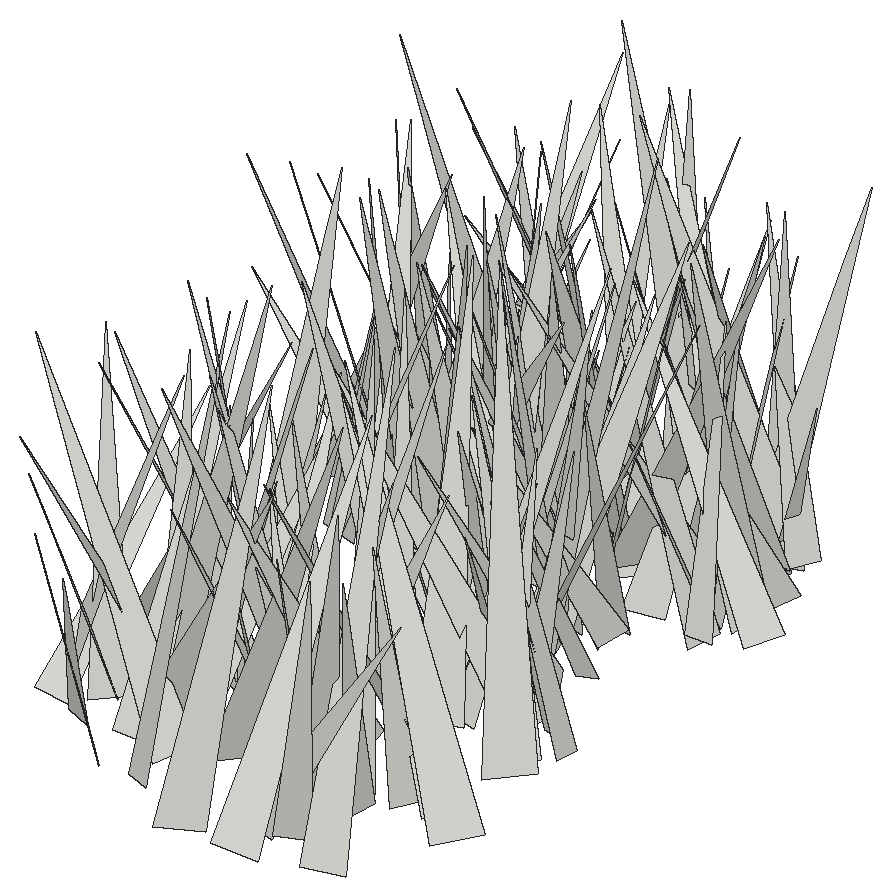
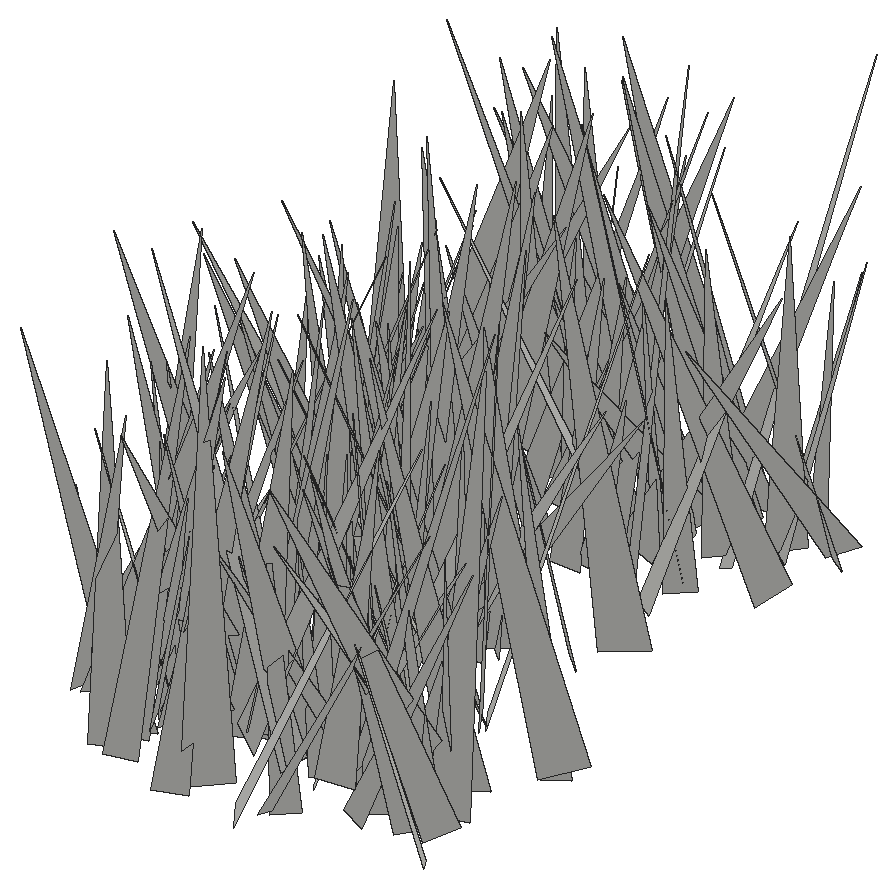
# SketchUp Ruby script. Lengths in inches.
U = 1.inch
M = Sketchup.active_model
def pt(a) = Geom::Point3d.new(a.map { |v| v * U })
def face(e, loops, mat)
  f = e.add_face(loops[0].map { |a| pt(a) })
  loops[1..].each { |l| e.add_face(l.map { |a| pt(a) }).erase! }
  f.material = f.back_material = mat if mat
  f
end
# faces: each face lists its corners as indices into pts; further lists are holes
def faces(e, pts, list, mat = nil) = list.each { |f| face(e, (f[0].is_a?(Array) ? f : [f]).map { |l| l.map { |i| pts[i] } }, mat) }
# xy, xz, yz: faces in a plane at the given z, y or x. An outline is a flat list of corners, or four numbers for a rectangle; further outlines are holes
def ring(l) = l.size == 4 ? [[l[0], l[1]], [l[2], l[1]], [l[2], l[3]], [l[0], l[3]]] : l.each_slice(2).to_a
def flat(e, list, mat, &to3) = list.each { |f| face(e, (f[0].is_a?(Array) ? f : [f]).map { |l| ring(l).map { |u, v| to3.(u, v) } }, mat) }
def xy(e, z, list, mat = nil) = flat(e, list, mat) { |x, y| [x, y, z] }
def xz(e, y, list, mat = nil) = flat(e, list, mat) { |x, z| [x, y, z] }
def yz(e, x, list, mat = nil) = flat(e, list, mat) { |y, z| [x, y, z] }
def lines(e, pts, list) = list.each { |a, b| e.add_line(pt(pts[a]), pt(pts[b])) }
# prism: a flat outline (further loops are holes) pulled along v
def prism(e, loops, v, mat = nil)
  f = face(e, loops, mat); d = Geom::Vector3d.new(v.map { |x| x * U })
  f.pushpull(f.normal.samedirection?(d) ? d.length : -d.length)
end
def box(e, o, s, mat = nil) = prism(e, [[o, [o[0] + s[0], o[1], o[2]], [o[0] + s[0], o[1] + s[1], o[2]], [o[0], o[1] + s[1], o[2]]]], [0, 0, s[2]], mat)
def at(x, y, z, deg = 0) = Geom::Transformation.translation(pt([x, y, z])) * Geom::Transformation.rotation(ORIGIN, Z_AXIS, deg.degrees)
def axes(o, x, y, z) = Geom::Transformation.new([*x, 0, *y, 0, *z, 0, *pt(o).to_a, 1])
def part(name) = M.definitions.add(name)
# library, detail: a bought-in or finely detailed component or shape, given as its bounding box
def library(name, o, s) = part(name).tap { |d| box(d.entities, o, s) }
def detail(e, o, s) = box(e.add_group.entities, o, s)
def put(e, d, t, mat = nil) = e.add_instance(d, t).tap { |i| i.material = mat if mat }
def group(e, t, mat = nil) = e.add_group.tap { |g| g.transformation = t; g.material = mat if mat }.entities
root = M.entities
c1 = part("fur_instance\#9")
p = [[0.8125,0,1.79],[0.67,-0.02,1.48],[0,-0.11,0],[0,0.11,0]]
faces(c1.entities,p,[[0,1,2,3]])
put(root,c1,axes([146.41,46.61,-27.1],[2.86346,-4.49186,1.0378],[-4.60706,-2.8331,0.44926],[-0.16992,1.11803,5.30796]))
put(root,c1,axes([138.79,46.7,-27.1],[-2.84095,-2.72325,0.75235],[-2.80656,2.8428,-0.30791],[0.32453,0.74533,3.9233]))
put(root,c1,axes([145.17,46.39,-27.1],[2.54302,-4.52945,1.06711],[-4.23804,-1.75205,2.66287],[1.92189,2.12978,4.46004]))
put(root,c1,axes([143.4,44.91,-27.1],[5.43285,-3.6045,3.64876],[-4.74936,-5.54221,1.59663],[-1.93634,3.48041,6.32132]))
put(root,c1,axes([136.69,48.41,-27.1],[-0.43336,-3.79274,0.22877],[-3.61563,0.48241,1.14868],[1.16807,0.08612,3.64049]))
put(root,c1,axes([137.43,51.93,-27.1],[-5.00279,-6.48805,0.18943],[-5.66686,4.48249,3.86684],[3.16501,-2.22958,7.22289]))
put(root,c1,axes([145.65,48.75,-27.1],[5.23742,-3.794,0.7561],[-3.79638,-5.28528,-0.22367],[-0.74406,0.26094,6.46336]))
put(root,c1,axes([145.58,44.87,-27.1],[-1.59566,7.05244,0.57454],[6.94745,1.67322,-1.24356],[1.34162,-0.27674,7.12297]))
put(root,c1,axes([146.96,49.14,-27.1],[4.83805,-1.95602,0.87332],[-1.75837,-4.85831,-1.14034],[-1.22345,-0.75248,5.09238]))
put(root,c1,axes([138.8,49.68,-27.1],[2.77166,-6.45652,0.14972],[-5.9267,-2.47813,2.8503],[2.56578,1.25036,6.42219]))
put(root,c1,axes([144.97,49.34,-27.1],[3.60771,1.96245,2.32029],[2.67745,-3.75626,-0.98607],[-1.43745,-2.07119,3.98679]))
put(root,c1,axes([140.375,48.45,-27.1],[-6.66331,2.16551,0.21128],[2.17487,6.60915,0.85019],[-0.06344,-0.87375,6.95459]))
put(root,c1,axes([136.41,50.5,-27.1],[-3.04266,-3.74721,0.50143],[-3.60797,3.07034,1.05183],[1.12942,-0.28668,4.71094]))
put(root,c1,axes([142.25,51.57,-27.1],[-3.9218,-4.42687,0.35438],[-4.07666,3.77609,2.05553],[1.7617,-1.11678,5.54549]))
put(root,c1,axes([148.41,45.6,-27.1],[0.0768,8.17284,0.16546],[8.06568,-0.10268,1.32775],[-1.3295,-0.15078,8.06464]))
put(root,c1,axes([141.87,49.24,-27.1],[6.48225,-3.39085,0.68777],[-3.4557,-6.41712,0.9323],[-0.17042,1.14593,7.25591]))
put(root,c1,axes([140.53,46.45,-27.1],[3.83849,6.3713,1.10198],[6.13828,-3.99344,1.70758],[-2.03209,-0.02789,7.23959]))
put(root,c1,axes([144.49,49.09,-27.1],[1.01992,4.1189,1.46608],[4.23417,-0.55549,-1.38501],[1.0893,-1.69737,4.0109]))
put(root,c1,axes([144.74,52.42,-27.1],[-6.04066,-0.63869,2.51357],[0.73038,5.69455,3.20222],[2.48847,-3.22176,5.16172]))
put(root,c1,axes([148.51,51.32,-27.1],[-2.23247,-5.83337,0.18602],[-5.6892,2.13065,-1.46288],[-1.30221,0.692,6.07224]))
put(root,c1,axes([142.72,50.27,-27.1],[-2.07432,-2.92088,0.84042],[-3.01146,2.11274,-0.09003],[0.41107,0.73854,3.58137]))
put(root,c1,axes([147.82,50.4,-27.1],[-3.6167,2.28369,2.19841],[2.80718,3.85669,0.61192],[1.47241,-1.74341,4.23336]))
put(root,c1,axes([144.92,50.83,-27.1],[1.50784,-3.41822,0.5063],[-3.4457,-1.52893,-0.06057],[-0.26023,0.4385,3.73552]))
put(root,c1,axes([143.4,52.11,-27.1],[1.95168,-6.84621,1.26966],[-6.52036,-2.2596,-2.16121],[-2.44285,0.56154,6.78298]))
put(root,c1,axes([144.15,50.15,-27.1],[4.85202,-3.37562,1.03104],[-3.52041,-4.75453,1.00059],[-0.25408,1.41409,5.82544]))
put(root,c1,axes([134.9,49.71,-27.1],[4.20289,4.66758,0.96744],[4.74909,-3.98911,-1.38552],[0.41036,-1.63927,6.12625]))
put(root,c1,axes([150.39,49.66,-27.1],[-4.97351,5.86998,1.15657],[5.9442,4.67754,1.82131],[-0.6788,-2.04794,7.47498]))
put(root,c1,axes([144.8,48.65,-27.1],[3.51205,7.24819,1.1392],[7.33442,-3.43356,-0.76524],[0.20101,-1.35755,8.01781]))
put(root,c1,axes([144.77,50.04,-27.1],[-7.94923,-1.56442,0.5472],[-1.62855,7.87073,-1.15603],[0.30767,1.24144,8.0188]))
put(root,c1,axes([139.36,51.0625,-27.1],[3.2608,1.42212,0.87051],[1.60342,-3.19897,-0.78016],[-0.45742,-1.07574,3.47082]))
put(root,c1,axes([136.67,49.96,-27.1],[-4.60516,3.74944,1.60687],[3.84875,4.79672,-0.16237],[1.35183,-0.88372,5.93628]))
put(root,c1,axes([140.39,49.5,-27.1],[4.26964,0.47793,1.18834],[0.14194,-4.28676,1.21405],[-1.27296,1.12502,4.1212]))
put(root,c1,axes([138.6,49.83,-27.1],[7.3545,-2.24014,2.18394],[-2.66673,-7.40612,1.38362],[-1.63595,2.00191,7.56257]))
put(root,c1,axes([144.25,50.67,-27.1],[2.31719,-2.3997,1.71249],[-2.74416,-2.55172,0.13746],[-1.07739,1.33819,3.33302]))
put(root,c1,axes([149.03,50.79,-27.1],[-5.22041,4.31379,0.87725],[4.39805,5.05275,1.32586],[-0.18846,-1.57859,6.64105]))
put(root,c1,axes([143.22,50.87,-27.1],[-3.14224,2.77876,1.0294],[2.91205,3.17344,0.32264],[0.54877,-0.92877,4.18224]))
put(root,c1,axes([138.76,48.47,-27.1],[0.11708,7.08162,0.20269],[7.08451,-0.11681,-0.01106],[0.00771,-0.20285,7.08258]))
put(root,c1,axes([146.03,50.17,-27.1],[0.42916,7.00561,1.64499],[7.11073,-0.66598,0.98114],[-1.10544,-1.56418,6.94983]))
put(root,c1,axes([135.26,48.95,-27.1],[-2.44099,4.81015,0.04297],[4.37742,2.2412,-2.21652],[1.99437,0.96814,4.91762]))
put(root,c1,axes([140.65,53.84,-27.1],[-0.18064,-6.52008,0.8881],[-6.57997,0.17015,-0.08916],[-0.06535,0.89016,6.52198]))
put(root,c1,axes([137.96,51.41,-27.1],[3.60386,-3.42869,2.87422],[-4.08632,-4.02533,0.32181],[-1.82182,2.24626,4.96388]))
put(root,c1,axes([138.57,55.16,-27.1],[-4.91582,-6.36103,2.07601],[-5.8042,5.33544,2.60426],[3.32923,-0.09063,7.60565]))
put(root,c1,axes([137.95,53.33,-27.1],[5.79589,4.16761,1.50359],[4.42839,-5.37215,-2.17978],[0.13803,-2.64446,6.79779]))
put(root,c1,axes([137.8125,55.41,-27.1],[-3.98509,-5.15803,0.00595],[-5.07141,3.91953,1.18509],[0.94137,-0.71992,6.40951]))
put(root,c1,axes([140.28,52.74,-27.1],[-1.81659,5.58818,1.87966],[5.39696,0.78429,2.88421],[-2.37355,-2.49359,5.11948]))
put(root,c1,axes([139.4,52.64,-27.1],[1.95895,3.98258,1.69888],[4.26762,-2.09086,-0.01944],[-0.73116,-1.53362,4.43825]))
put(root,c1,axes([135.21,52.4,-27.1],[6.85637,-0.90607,0.05149],[-0.90407,-6.7849,0.99057],[0.07926,0.98874,6.84468]))
put(root,c1,axes([139.62,50.28,-27.1],[-3.68567,4.23937,0.30212],[3.60627,3.33103,-2.74713],[2.24908,1.60613,4.89997]))
put(root,c1,axes([137.53,53.98,-27.1],[-2.45808,3.26284,2.53045],[3.74921,2.99751,-0.22312],[1.72995,-1.86016,4.07903]))
put(root,c1,axes([141.08,51.95,-27.1],[-2.87102,4.68172,0.40163],[4.57171,2.89185,-1.02921],[1.08596,0.20316,5.39463]))
put(root,c1,axes([142.53,54.32,-27.1],[1.52627,-4.48364,1.33128],[-4.39877,-0.90019,2.01128],[1.58937,1.81423,4.28804]))
put(root,c1,axes([141.25,54.89,-27.1],[0.46643,-4.66615,1.44002],[-4.86096,-0.58186,-0.31092],[-0.46655,1.39737,4.67909]))
put(root,c1,axes([144.375,55.51,-27.1],[4.0303,-5.81988,3.12764],[-5.66664,-4.92868,-1.86917],[-3.39741,1.31665,6.82792]))
put(root,c1,axes([149.18,53.7,-27.1],[-6.71454,4.39928,1.56364],[4.39375,6.8803,-0.4901],[1.57912,-0.43767,8.0124]))
put(root,c1,axes([147.71,56.43,-27.1],[-4.43221,4.72995,1.58971],[4.78005,3.41433,3.16821],[-1.43205,-3.24253,5.65503]))
put(root,c1,axes([140.52,54.53,-27.1],[-1.14245,4.14217,0.46464],[4.01441,0.96381,1.27839],[-1.12161,-0.76952,4.10226]))
put(root,c1,axes([140.23,53.22,-27.1],[5.64336,5.1887,0.30355],[5.15395,-5.64438,0.66329],[-0.67191,0.28398,7.63742]))
put(root,c1,axes([148.5625,56.52,-27.1],[-1.63509,-3.83691,0.93062],[-3.94815,1.58786,-0.39017],[-0.00453,1.00909,4.15248]))
put(root,c1,axes([145.66,57.87,-27.1],[-0.82646,-4.24361,0.01629],[-4.06802,0.79698,1.2278],[1.20816,-0.21938,4.14533]))
put(root,c1,axes([148.79,54.63,-27.1],[-4.40287,4.25609,0.42122],[4.26988,4.40886,0.08361],[0.24458,-0.35298,6.12311]))
put(root,c1,axes([146.87,58.99,-27.1],[-4.92711,-3.11526,0.5387],[-2.69685,4.66208,2.29422],[1.64986,-1.68274,5.3589]))
put(root,c1,axes([148.49,54.45,-27.1],[-4.43133,1.84787,0.51045],[1.62369,4.30117,-1.47494],[1.01922,1.18203,4.56901]))
put(root,c1,axes([145.41,54.89,-27.1],[-2.63415,6.93544,1.64719],[7.09873,2.71215,-0.06728],[0.64926,-1.51533,7.41852]))
put(root,c1,axes([147.15,56.875,-27.1],[-4.76846,2.17787,1.48985],[2.383,4.8757,0.4998],[1.13316,-1.08876,5.21838]))
put(root,c1,axes([149.72,55.79,-27.1],[-6.70794,-1.60484,0.19836],[-1.59675,6.44001,-1.8942],[-0.25542,1.88735,6.63204]))
put(root,c1,axes([137.375,56.8125,-27.1],[1.77196,3.84512,1.4323],[4.08534,-1.50774,-1.0065],[0.38272,-1.70823,4.11239]))
put(root,c1,axes([146.46,57.375,-27.1],[0.92533,-3.44435,1.34936],[-3.58141,-1.18238,-0.56215],[-0.92618,1.13092,3.52189]))
put(root,c1,axes([143.45,55.51,-27.1],[-0.40472,6.25604,0.83945],[6.18781,0.22712,1.29072],[-1.24649,-0.90382,6.13481]))
put(root,c1,axes([145.23,56.27,-27.1],[3.77133,0.16267,0.95437],[-0.10228,-3.74984,1.04331],[-0.96272,1.03561,3.6278]))
put(root,c1,axes([144.08,59.74,-27.1],[4.85347,-3.26157,0.26621],[-3.0891,-4.72355,-1.55255],[-1.07988,-1.1468,5.6377]))
put(root,c1,axes([146.98,57.32,-27.1],[4.06657,-2.17936,1.39694],[-2.40276,-4.14574,0.52683],[-0.9632,1.14071,4.58356]))
put(root,c1,axes([145.72,55.51,-27.1],[2.14003,7.20036,0.0672],[7.19519,-2.14104,0.27303],[-0.28086,0.01341,7.50668]))
put(root,c1,axes([136.58,57.83,-27.1],[-2.68799,6.56885,2.98447],[6.8694,3.30396,-1.08507],[2.20641,-2.2839,7.01411]))
put(root,c1,axes([141.82,59.57,-27.1],[7.52805,-0.18805,1.99939],[0.07054,-7.72753,-0.99239],[-2.00698,-0.97696,7.46472]))
put(root,c1,axes([143.22,60.36,-27.1],[-6.0404,2.2493,3.21945],[3.13358,6.3206,1.46334],[2.36747,-2.62704,6.2773]))
put(root,c1,axes([147.16,59.96,-27.1],[-0.83843,-4.56243,0.7415],[-4.45874,0.59959,-1.35228],[-1.2187,0.94513,4.43735]))
put(root,c1,axes([144.71,57.46,-27.1],[-3.134,4.47853,0.59876],[4.43295,3.18866,-0.64743],[0.8745,-0.1137,5.42771]))
put(root,c1,axes([140.36,61.11,-27.1],[1.08245,-7.41016,1.80762],[-7.58562,-1.23679,-0.52762],[-0.7977,1.70574,7.47019]))
put(root,c1,axes([141.34,61.09,-27.1],[1.42395,-7.42701,2.10024],[-7.62151,-1.69014,-0.80943],[-1.21824,1.89264,7.51884]))
put(root,c1,axes([146.28,62.32,-27.1],[3.38656,-3.48151,1.0277],[-2.77448,-3.38882,-2.33752],[-2.3408,-1.02022,4.25743]))
put(root,c1,axes([139.91,60.01,-27.1],[-4.37552,-5.12362,2.64469],[-5.63456,4.50416,-0.59611],[1.22377,2.41912,6.71129]))
put(root,c1,axes([145.33,60.91,-27.1],[-6.26815,-2.22604,2.13273],[-2.17784,6.6177,0.5065],[2.18193,0.21043,6.63238]))
put(root,c1,axes([140.89,60.79,-27.1],[-3.83855,4.56526,0.77541],[4.17711,2.97899,3.13921],[-1.99865,-2.54191,5.07163]))
put(root,c1,axes([137.43,59.3,-27.1],[2.58432,3.47984,0.90101],[3.42396,-2.72089,0.68775],[-1.09434,-0.29537,4.2796]))
put(root,c1,axes([145.52,58.74,-27.1],[6.4283,2.09347,0.22673],[2.03253,-6.35917,1.08941],[-0.55031,0.96716,6.67224]))
put(root,c1,axes([145.21,60.52,-27.1],[5.91491,-0.67607,1.90084],[-0.77835,-6.19702,0.21795],[-1.8613,0.44302,5.94943]))
put(root,c1,axes([145.85,62.93,-27.1],[0.34868,-5.31048,0.36463],[-5.26358,-0.28954,0.81646],[0.79301,0.41316,5.25892]))
put(root,c1,axes([137.14,63.8,-27.1],[-6.21102,-4.85766,0.88936],[-4.64444,6.23147,1.60082],[1.67841,-0.73247,7.72082]))
put(root,c1,axes([144.45,64.03,-28.22],[-6.5639,-4.29471,0.69968],[-4.06333,6.50273,1.7952],[1.55674,-1.13527,7.63588]))
put(root,c1,axes([141.12,60.06,-27.1],[-6.11447,-3.98639,0.59028],[-3.68819,5.10346,-3.73879],[-1.62389,3.41906,6.26894]))
put(root,c1,axes([143.76,60.29,-27.1],[-4.22823,5.63878,0.60494],[5.64653,4.11564,1.10357],[-0.52773,-1.14251,6.96102]))
put(root,c1,axes([144.16,63.45,-27.1],[-4.57132,-4.01454,0.83204],[-3.89365,4.6413,1.00178],[1.28384,-0.21818,6.00082]))
put(root,c1,axes([138.18,63.78,-27.1],[1.13503,-7.67663,0.6742],[-6.50823,-0.58999,4.2389],[4.12651,1.18099,6.50005]))
put(root,c1,axes([139.35,59.78,-27.1],[-4.20767,6.2047,0.57896],[6.20765,4.23458,-0.26697],[0.54635,-0.32858,7.49209]))
put(root,c1,axes([144.33,59.26,-27.1],[3.4696,4.95294,0.18512],[4.68916,-3.35343,1.83583],[-1.60551,0.90933,5.7619]))
put(root,c1,axes([141.11,62.59,-27.1],[5.21956,1.10973,1.69595],[1.36173,-5.39042,-0.66376],[-1.50115,-1.03121,5.29478]))
put(root,c1,axes([140.17,64.52,-27.1],[-4.57477,-6.03245,0.25242],[-6.03633,4.57654,-0.02819],[0.13005,0.21817,7.57088]))
put(root,c1,axes([146.06,58.62,-27.1],[7.29611,1.84526,3.54482],[-0.04664,-7.33917,3.91643],[-3.99607,3.45479,6.4265]))
put(root,c1,axes([134.5,63.76,-28.22],[0.54307,-5.39112,1.14857],[-5.29865,-0.1925,1.60174],[1.51911,1.25582,5.17624]))
put(root,c1,axes([140.59,63.66,-28.22],[6.72646,1.81373,2.96578],[2.30607,-7.16166,-0.85049],[-2.60144,-1.65881,6.91459]))
put(root,c1,axes([144.55,61.13,-27.1],[-2.83058,6.09964,1.95872],[5.76034,3.3604,-2.14023],[2.80369,-0.74599,6.37473]))
put(root,c1,axes([142.11,64.96,-27.1],[2.97455,-6.14482,0.55918],[-6.16848,-2.94679,0.43089],[0.14598,0.69067,6.8133]))
put(root,c1,axes([140.75,63.15,-27.1],[1.70203,4.17643,2.24286],[4.55719,-2.09788,0.44817],[-1.30578,-1.87783,4.48761]))
put(root,c1,axes([143.98,62.23,-27.1],[0.03547,5.69131,1.501],[5.73382,0.30561,-1.29426],[1.32938,-1.46999,5.5423]))
put(root,c1,axes([144.48,62.46,-27.1],[-6.24639,-1.28271,0.8155],[-1.43317,6.11916,-1.35263],[0.50635,1.49608,6.23162]))
put(root,c1,axes([141.22,64.93,-27.1],[5.81845,-0.62274,2.18855],[-0.03101,-6.03017,-1.6334],[-2.27522,-1.51035,5.61909]))
put(root,c1,axes([141.76,63.3,-27.1],[-3.37291,-1.64413,0.77782],[-1.79286,3.28135,-0.83849],[0.30629,1.10194,3.65741]))
put(root,c1,axes([141.93,61.83,-27.1],[-0.24232,8.0833,1.63068],[8.24361,0.27788,-0.15248],[0.20433,-1.625,8.08549]))
put(root,c1,axes([137.36,63.79,-27.1],[-5.46878,-3.64969,2.6695],[-4.02035,5.84198,-0.2491],[2.0696,1.70441,6.57007]))
put(root,c1,axes([137.02,65.34,-28.22],[5.21183,-0.69159,1.00189],[-0.40075,-5.13378,-1.45906],[-1.14955,-1.3458,5.051]))
put(root,c1,axes([138.2,63.49,-28.22],[3.11612,2.14822,0.04863],[2.13222,-3.08072,-0.53874],[0.26618,-0.47091,3.74631]))
put(root,c1,axes([133.34,64.82,-27.1],[5.01421,-5.55154,0.43768],[-5.45899,-4.78379,1.86233],[1.10028,1.565,7.24525]))
put(root,c1,axes([146.52,67.51,-28.22],[-6.99156,-3.62516,0.34789],[-3.32905,6.6672,2.57109],[1.47657,-2.13338,7.444]))
put(root,c1,axes([143.4,63.27,-27.1],[3.40494,2.47984,0.75094],[2.39973,-3.48584,0.63038],[-0.97714,0.08048,4.16483]))
put(root,c1,axes([143.88,63.54,-28.22],[2.11114,4.26728,1.69749],[4.08085,-2.60007,1.46097],[-2.10662,-0.76029,4.53125]))
put(root,c1,axes([137.3,63.77,-27.1],[4.92095,5.18553,0.33695],[5.09859,-4.72846,-1.69263],[1.00379,-1.4039,6.94554]))
put(root,c1,axes([148,64.83,-27.1],[-3.22375,-2.36609,0.00506],[-2.25529,3.0702,-1.21594],[-0.71558,0.9831,3.80952]))
put(root,c1,axes([139.46,65.26,-27.1],[-0.7765,-5.95979,2.50914],[-6.25232,1.3369,1.24057],[1.65027,2.26084,5.88073]))
put(root,c1,axes([148.35,63.86,-27.1],[0.28645,5.00767,1.03913],[5.08565,-0.389,0.47271],[-0.54104,-1.00525,4.99354]))
put(root,c1,axes([143.35,65.36,-28.22],[5.91305,2.63208,1.30513],[2.84881,-5.85376,-1.10147],[-0.71801,-1.54954,6.37799]))
put(root,c1,axes([141.27,64.5625,-27.1],[1.148,3.43718,0.90942],[3.54891,-1.0498,-0.51218],[0.21566,-1.0212,3.58745]))
put(root,c1,axes([149.99,65.01,-27.1],[-4.53112,4.00144,0.54603],[3.94801,4.21612,1.86503],[-0.85024,-1.74745,5.75015]))
put(root,c1,axes([142.72,66.98,-27.1],[-2.91514,-5.53327,1.42514],[-5.42873,3.18122,1.24695],[1.78243,0.63944,6.12864]))
put(root,c1,axes([141.09,66.24,-27.1],[3.87563,-0.57439,1.14349],[-0.32332,-3.96837,-0.89752],[-1.23813,-0.76168,3.81378]))
put(root,c1,axes([140.42,65.34,-28.22],[4.6292,0.17151,0.50537],[0.17521,-4.6565,-0.02456],[-0.5041,-0.0434,4.63231]))
put(root,c1,axes([147.22,67.36,-27.1],[1.68994,-6.65431,0.98946],[-6.7239,-1.70391,0.02495],[-0.21912,0.96522,6.8655]))
put(root,c1,axes([135.6,67.6,-28.22],[0.64901,-7.30772,0.94418],[-7.33385,-0.54888,0.79295],[0.71332,1.00569,7.2935]))
put(root,c1,axes([140.78,65.02,-28.22],[-0.2633,5.21725,2.01289],[5.21535,0.95622,-1.79623],[2.01778,-1.79073,4.90536]))
put(root,c1,axes([141.66,68.48,-27.1],[5.49992,-4.64771,0.52674],[-4.40214,-5.41809,-1.84207],[-1.58109,-1.08206,6.96111]))
put(root,c1,axes([137.22,67.37,-28.22],[3.42862,-3.42654,1.21049],[-3.04602,-3.61734,-1.61199],[-1.98197,-0.36822,4.57144]))
put(root,c1,axes([147.3,65.43,-28.22],[-7.05219,-0.0174,0.36445],[-0.04272,7.04446,-0.49029],[0.36236,0.49184,7.03515]))
put(root,c1,axes([139.93,68.65,-28.22],[-4.13321,-3.41194,0.20507],[-3.07913,3.85633,2.10107],[1.48403,-1.5014,4.93054]))
put(root,c1,axes([143.77,66.04,-27.1],[7.07032,-2.50038,0.22823],[-2.5064,-6.98854,1.08245],[0.14815,1.09629,7.42089]))
put(root,c1,axes([140.6,66.37,-28.22],[-3.23089,-3.2407,0.20186],[-3.09319,2.98531,-1.58167],[-0.98745,1.25194,4.29408]))
put(root,c1,axes([136.15,65.92,-28.22],[1.86303,-6.4471,2.90273],[-6.99316,-1.23765,1.73947],[1.04242,3.21946,6.48153]))
put(root,c1,axes([143.08,67.04,-27.1],[-3.69542,-5.95234,1.80806],[-6.20183,3.68953,-0.52934],[0.48649,1.82006,6.98615]))
put(root,c1,axes([148.42,67.03,-28.22],[-2.94659,-4.28728,0.79485],[-4.35538,2.84813,-0.78348],[-0.2081,1.09651,5.14289]))
put(root,c1,axes([146.64,66.4375,-27.1],[-2.09497,-3.98677,2.51489],[-4.46346,2.56262,0.34425],[1.51546,2.03632,4.49052]))
put(root,c1,axes([137.96,65.73,-27.1],[3.6626,3.70148,0.35684],[3.71844,-3.64024,-0.40601],[0.03906,-0.53912,5.19141]))
put(root,c1,axes([138.32,65.73,-28.22],[2.93854,2.24557,1.05284],[2.03507,-3.11619,0.96641],[-1.41759,0.18132,3.56983]))
put(root,c1,axes([147.68,66.89,-28.22],[-4.77809,0.40303,0.49366],[0.4272,4.79644,0.21897],[0.47289,-0.2608,4.79006]))
put(root,c1,axes([141.6,67.73,-27.1],[5.62437,-1.82953,0.08499],[-1.8284,-5.62476,-0.0835],[-0.10665,-0.05312,5.91386]))
put(root,c1,axes([147.75,68.84,-28.22],[2.95419,-3.46444,1.08183],[-2.95275,-3.10527,-1.88109],[-2.11044,-0.50488,4.14621]))
put(root,c1,axes([141.02,66.91,-28.22],[1.67153,-3.68103,1.97281],[-4.08391,-1.88531,-0.05752],[-0.87388,1.76964,4.04237]))
put(root,c1,axes([136.32,66.71,-28.22],[2.05844,3.54151,1.67651],[3.74882,-2.33096,0.32115],[-1.13989,-1.27062,4.08367]))
put(root,c1,axes([138.6,65.73,-28.22],[1.45638,3.8911,0.37542],[3.87774,-1.48869,0.38679],[-0.49475,-0.21394,4.13668]))
put(root,c1,axes([142.1,69.19,-27.1],[-4.63636,-6.55031,0.51962],[-6.56307,4.58532,-0.75728],[-0.32055,0.86066,7.9893]))
put(root,c1,axes([138.32,68.51,-27.1],[-7.66466,-1.90179,1.421],[-1.79066,7.78455,0.75987],[1.55871,-0.40873,7.86043]))
put(root,c1,axes([147.3125,68.85,-27.1],[-0.33805,-5.61743,0.95415],[-5.65981,0.22074,-0.70569],[-0.6576,0.9879,5.58317]))
put(root,c1,axes([136.26,67.48,-28.22],[2.41252,4.65389,1.89869],[5.02303,-2.30836,-0.72433],[-0.1815,-2.02404,5.19175]))
put(root,c1,axes([140.15,68.07,-28.22],[0.50859,-3.54434,0.97529],[-3.61365,-0.30136,0.78924],[0.67458,1.05784,3.49258]))
put(root,c1,axes([137.42,68.73,-28.22],[0.50493,-3.90237,0.56248],[-3.75126,-0.30094,1.27958],[1.21364,0.69337,3.72104]))
put(root,c1,axes([146.99,68.09,-27.1],[-2.52237,2.99386,0.77548],[2.99232,2.10973,1.58806],[-0.78138,-1.58517,3.57821]))
put(root,c1,axes([143.84,68.22,-28.22],[6.74375,-1.56753,0.95704],[-1.61805,-6.79399,0.27364],[-0.86892,0.48558,6.91813]))
put(root,c1,axes([142.55,66.68,-28.22],[1.32341,3.79294,0.4756],[3.74321,-1.38791,0.65276],[-0.77522,-0.22654,3.9638]))
put(root,c1,axes([143.74,70.31,-28.22],[-4.79038,-5.44103,1.36632],[-5.2062,4.98101,1.5825],[2.08977,-0.06337,7.07448]))
put(root,c1,axes([137.79,69.4375,-28.22],[-1.33885,-4.31341,0.19295],[-4.24788,1.27969,-0.86785],[-0.77346,0.43835,4.43226]))
put(root,c1,axes([137.4,68.46,-27.1],[4.80931,3.10321,2.02961],[3.46778,-4.94111,-0.66234],[-1.31293,-1.68352,5.68513]))
put(root,c1,axes([145.71,68.34,-28.22],[0.99186,4.25892,2.03749],[4.71935,-0.95274,-0.30591],[-0.13232,-2.05608,4.36218]))
put(root,c1,axes([143.3,67.41,-28.22],[-4.74257,5.72398,1.5327],[5.90767,4.72004,0.65254],[0.46105,-1.60076,7.40474]))
put(root,c1,axes([147.29,69.46,-27.1],[-7.26006,2.55391,1.83228],[2.95803,7.11093,1.80912],[1.0629,-2.34529,7.48051]))
put(root,c1,axes([144.82,65.61,-28.22],[-4.70627,4.28235,1.06672],[3.70191,4.67966,-2.45399],[2.40255,1.178,5.87073]))
put(root,c1,axes([143.54,68.06,-27.1],[4.7353,0.6555,1.15241],[0.55235,-4.8611,0.49538],[-1.20525,0.34759,4.75472]))
put(root,c1,axes([138.68,67.43,-28.22],[0.32449,4.79651,0.65441],[4.29347,0.01783,-2.25961],[2.23626,-0.73022,4.24334]))
put(root,c1,axes([140.02,69.49,-27.1],[8.09633,1.85359,0.38508],[1.89305,-7.94545,-1.5559],[-0.02113,-1.6027,8.15877]))
put(root,c1,axes([144.97,70.02,-27.1],[-5.38028,-3.08502,1.66928],[-3.07413,5.61908,0.47644],[1.68926,0.39986,6.18367]))
put(root,c1,axes([146.23,67.74,-27.1],[3.62964,3.56201,0.97293],[3.43547,-3.75775,0.94107],[-1.35352,0.01415,4.99765]))
put(root,c1,axes([139.58,70.43,-28.22],[2.72527,-3.47225,0.02549],[-3.46346,-2.7159,0.33551],[0.24824,0.22715,4.40125]))
put(root,c1,axes([138.33,69.62,-27.1],[1.39978,-5.30319,2.32473],[-5.64349,-1.78474,-0.67328],[-1.29585,2.04412,5.44334]))
put(root,c1,axes([146.63,69.91,-28.22],[3.71508,-1.29272,0.27873],[-1.28155,-3.72443,-0.19222],[-0.32626,-0.0905,3.92887]))
put(root,c1,axes([135.88,68.85,-28.22],[3.16186,-4.77933,2.12939],[-5.21892,-2.70344,1.68164],[0.37303,2.68757,5.47827]))
put(root,c1,axes([136.93,65.98,-28.22],[5.40862,3.75774,0.29196],[3.28966,-4.95573,2.84217],[-1.83956,2.18614,5.94103]))
put(root,c1,axes([144.36,72.4,-27.1],[-0.43827,-6.52973,0.002],[-6.42899,0.43186,1.145],[1.14256,-0.07472,6.44348]))
put(root,c1,axes([133.84,70.0625,-27.1],[3.57334,-4.4658,0.19156],[-4.12422,-3.19939,2.34597],[1.72363,1.60293,5.21618]))
put(root,c1,axes([146.41,68.3125,-27.1],[-6.04879,4.39479,0.23194],[4.40071,6.03643,0.38865],[-0.04117,-0.45072,7.46666]))
put(root,c1,axes([144.76,71.1875,-27.1],[1.52104,-3.59534,0.18519],[-3.58042,-1.53172,-0.32978],[-0.37596,0.04131,3.88989]))
put(root,c1,axes([144.45,69.35,-27.1],[-8.05212,1.79962,1.36323],[1.82873,8.16018,0.02927],[1.32393,-0.32629,8.25072]))
put(root,c1,axes([140.72,71.45,-28.22],[-5.75391,-4.14909,0.07824],[-4.14913,5.75437,0.02082],[0.07564,0.02888,7.0938]))
put(root,c1,axes([146.48,67.74,-27.1],[-5.7713,0.32455,0.04644],[0.28097,5.31808,-2.2482],[0.16895,2.24233,5.3253]))
put(root,c1,axes([141.24,67.33,-28.22],[-5.90287,3.96424,1.22936],[3.5461,5.92766,-2.08769],[2.15678,1.10365,6.7971]))
put(root,c1,axes([134.35,70.26,-28.22],[4.18709,2.7222,0.51054],[2.74144,-3.94162,-1.4666],[0.39441,-1.502,4.77401]))
put(root,c1,axes([136.74,66.42,-28.22],[-5.0261,5.87636,0.71878],[5.2638,4.86732,-2.98524],[2.70938,1.44485,7.13314]))
put(root,c1,axes([143.11,71.6,-28.22],[2.7716,-4.32676,0.73791],[-4.29866,-2.85215,-0.57784],[-0.88707,0.30254,5.10575]))
put(root,c1,axes([138.86,72.33,-27.1],[-4.92347,-1.39259,0.14711],[-1.23579,4.5738,1.93769],[0.65861,-1.82825,4.73553]))
put(root,c1,axes([146.26,70.51,-28.22],[-1.98157,5.41612,3.08152],[6.10168,2.34277,-0.19399],[1.26474,-2.81671,5.76397]))
put(root,c1,axes([147.97,69.42,-27.1],[-5.43325,1.77797,0.85582],[1.73658,5.49897,-0.39929],[0.93695,0.1182,5.7028]))
put(root,c1,axes([146.22,69.27,-28.22],[0.16131,6.95669,2.04491],[7.08472,0.28432,-1.5261],[1.54396,-2.03146,6.78915]))
put(root,c1,axes([142.51,70.51,-28.22],[5.17413,-4.7343,3.23528],[-5.24163,-5.67192,0.08293],[-2.32507,2.25121,7.01272]))
